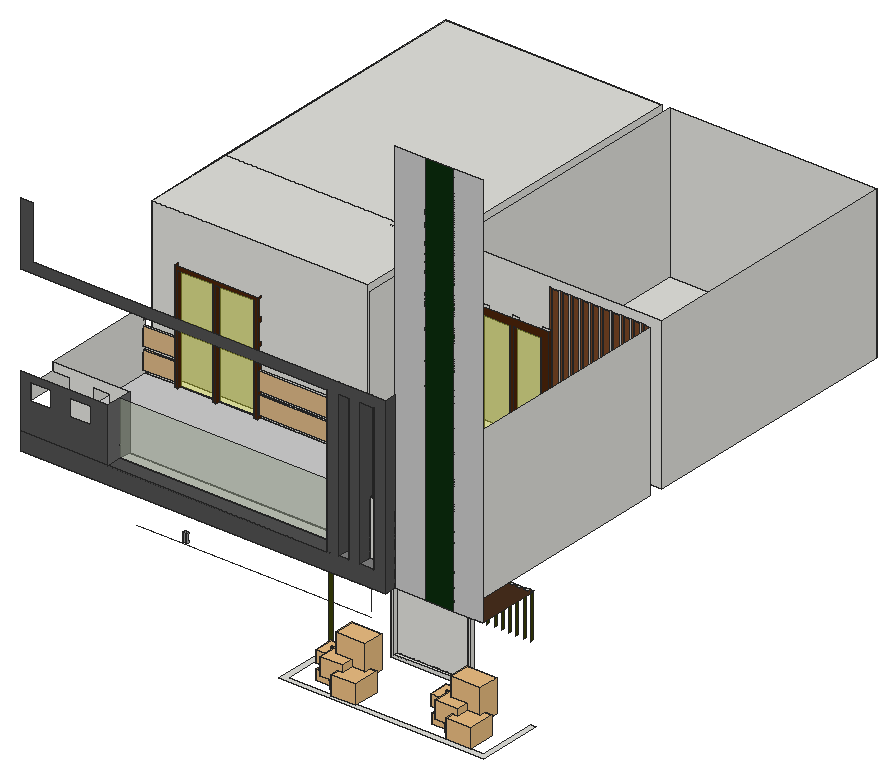
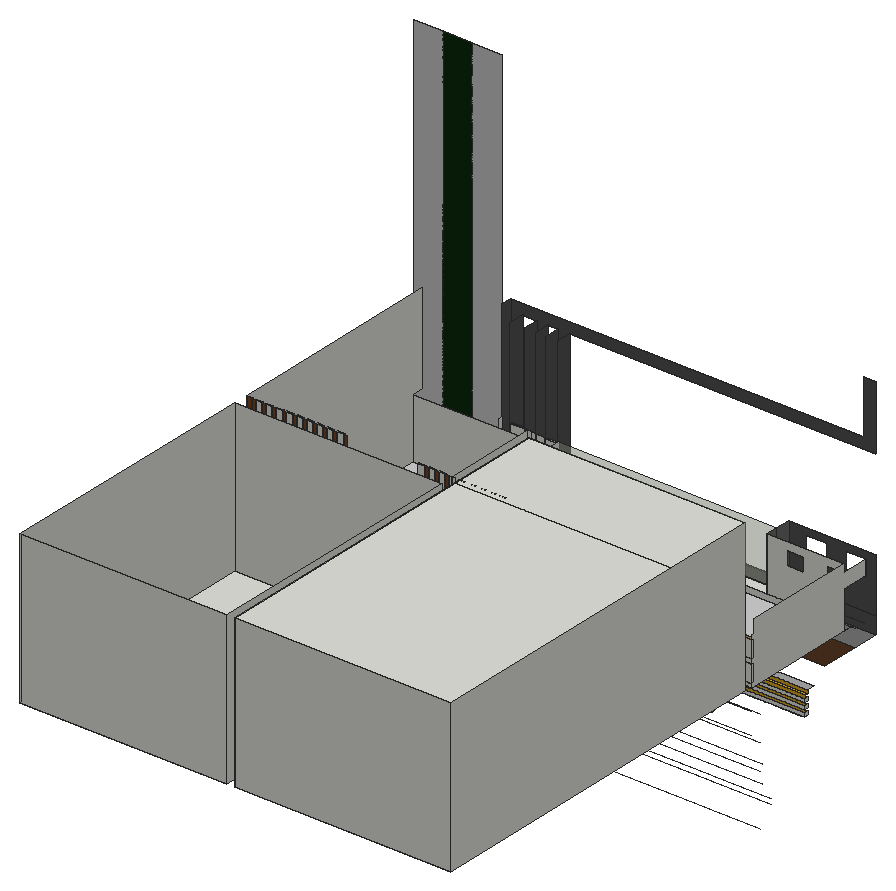
# SketchUp Ruby script. Lengths in inches.
U = 1.inch
M = Sketchup.active_model
def pt(a) = Geom::Point3d.new(a.map { |v| v * U })
def face(e, loops, mat)
  f = e.add_face(loops[0].map { |a| pt(a) })
  loops[1..].each { |l| e.add_face(l.map { |a| pt(a) }).erase! }
  f.material = f.back_material = mat if mat
  f
end
# faces: each face lists its corners as indices into pts; further lists are holes
def faces(e, pts, list, mat = nil) = list.each { |f| face(e, (f[0].is_a?(Array) ? f : [f]).map { |l| l.map { |i| pts[i] } }, mat) }
# xy, xz, yz: faces in a plane at the given z, y or x. An outline is a flat list of corners, or four numbers for a rectangle; further outlines are holes
def ring(l) = l.size == 4 ? [[l[0], l[1]], [l[2], l[1]], [l[2], l[3]], [l[0], l[3]]] : l.each_slice(2).to_a
def flat(e, list, mat, &to3) = list.each { |f| face(e, (f[0].is_a?(Array) ? f : [f]).map { |l| ring(l).map { |u, v| to3.(u, v) } }, mat) }
def xy(e, z, list, mat = nil) = flat(e, list, mat) { |x, y| [x, y, z] }
def xz(e, y, list, mat = nil) = flat(e, list, mat) { |x, z| [x, y, z] }
def yz(e, x, list, mat = nil) = flat(e, list, mat) { |y, z| [x, y, z] }
def lines(e, pts, list) = list.each { |a, b| e.add_line(pt(pts[a]), pt(pts[b])) }
# prism: a flat outline (further loops are holes) pulled along v
def prism(e, loops, v, mat = nil)
  f = face(e, loops, mat); d = Geom::Vector3d.new(v.map { |x| x * U })
  f.pushpull(f.normal.samedirection?(d) ? d.length : -d.length)
end
def box(e, o, s, mat = nil) = prism(e, [[o, [o[0] + s[0], o[1], o[2]], [o[0] + s[0], o[1] + s[1], o[2]], [o[0], o[1] + s[1], o[2]]]], [0, 0, s[2]], mat)
def at(x, y, z, deg = 0) = Geom::Transformation.translation(pt([x, y, z])) * Geom::Transformation.rotation(ORIGIN, Z_AXIS, deg.degrees)
def axes(o, x, y, z) = Geom::Transformation.new([*x, 0, *y, 0, *z, 0, *pt(o).to_a, 1])
def part(name) = M.definitions.add(name)
# library, detail: a bought-in or finely detailed component or shape, given as its bounding box
def library(name, o, s) = part(name).tap { |d| box(d.entities, o, s) }
def detail(e, o, s) = box(e.add_group.entities, o, s)
def put(e, d, t, mat = nil) = e.add_instance(d, t).tap { |i| i.material = mat if mat }
def group(e, t, mat = nil) = e.add_group.tap { |g| g.transformation = t; g.material = mat if mat }.entities
root = M.entities
M.materials.add("Material__1").color = [95, 70, 46]
M.materials.add("Material__2").color = [150, 168, 104]
M.materials.add("Material__3").color = [234, 233, 231]
M.materials.add("Material__4").color = [36, 36, 36]
M.materials.add("Material__5").color = [151, 172, 33]
M.materials.add("Material__6").color = [79, 108, 5]
M.materials.add("[0036_BurlyWood]").color = [222, 184, 135]
M.materials.add("[0043_SaddleBrown]1").color = [58, 63, 9]
M.materials.add("[0043_SaddleBrown]2").color = [76, 37, 10]
M.materials.add("[0045_Goldenrod]").color = [218, 165, 32]
M.materials.add("[0132_LightGray]").color = [169, 169, 169]
M.materials.add("[0133_Gray]").color = [128, 128, 128]
M.materials.add("[0134_DimGray]").color = [105, 105, 105]
M.materials.add("[0135_DarkGray]").color = [81, 81, 81]
M.materials.add("[Beadboard]").color = [71, 46, 29]
M.materials.add("[Carrera Marble]").color = [207, 207, 207]
M.materials.add("[Checker Plate]").color = [201, 201, 201]
M.materials.add("[Color M05]").color = [114, 114, 114]
M.materials.add("[Herringbone 4x1]").color = [12, 45, 14]
M.materials.add("[Polished Concrete Old]").color = [168, 168, 168]
M.materials.add("[Translucent Glass Blue]").color = [178, 191, 166]
M.materials["[Translucent Glass Blue]"].alpha = 0.5
M.materials.add("[Translucent Glass Gray]").color = [209, 214, 54]
M.materials["[Translucent Glass Gray]"].alpha = 0.5
M.materials.add("[Wood Veneer 01]").color = [120, 70, 37]
M.materials.add("wire_1").color = [140, 184, 58]
M.materials.add("wire_2").color = [244, 244, 244]
M.materials.add("wire_4").color = [86, 225, 198]
M.materials.add("wire_5").color = [232, 232, 232]
c1 = library("Group\#1",[-915.9375,-34.5,735.6],[41.04,40.85,6.81])
c2 = library("Group\#2",[-991.92,-34.05,729.49],[10.64,7.28,57.53])
c3 = library("Group\#3",[-1022.2,-71.69,736.68],[86.94,78.77,45.64])
c4 = library("Group\#4",[-877.77,-100.41,669.81],[37.9,37.9,42.75])
c5 = library("Group\#5",[-957.79,-83.08,701.98],[44.29,44.29,27.78])
c6 = library("Group\#6",[-1023.9,-65.47,669.625],[67.53,67.55,39.17])
c7 = library("Group\#7",[-997.48,-49.45,708.79],[29.81,29.81,30.61])
c8 = library("Group\#8",[-956738.95,-82059.81,669752.625],[42194.58,42232.57,49521.48])
c9 = library("Group\#9",[-917.52,-36.6875,711.84],[44.99,44.98,28.22])
c10 = library("Group\#10",[-916244.63,-35413.97,669800.48],[42442.38,42642.99,59706.29])
c11 = library("Group\#11",[-955.48,-54.29,730.4],[118.63,83.7,130.4])
c12 = library("Group\#12",[-899.97,-18.72,732.17],[8.78,8.27,28.64])
c13 = library("Group\#13",[-906.16,-138.28,686.8],[98.25,106.18,75.79])
c14 = library("Group\#14",[-978.71,-103.24,719.12],[90.2,76.4,68.29])
c15 = library("Group\#15",[-955.98,-81.17,725.57],[41.03,40.85,6.81])
c16 = library("Group\#16",[-996.8,-48.73,736.67],[28.51,28.38,4.73])
c17 = library("Group\#17",[-876.58,-99.29,706.19],[35.74,35.58,5.93])
c18 = library("Group\#18",[-912.1,-32.49,735.82],[33.14,36.63,9.55])
c19 = library("Group\#19",[-994.36,-46.95,735.88],[24.38,25.9,6.88])
c20 = part("PLANT-30")
p = [[0,0,0],[1,0,0],[1,1,0]]
lines(c20.entities,p,[[0,1],[1,2],[2,0]])
put(c20.entities,c1,at(895.63,-7.06,-669.82),"Material__1")
put(c20.entities,c2,at(895.63,-7.06,-669.82),"wire_1")
put(c20.entities,c3,at(895.63,-7.06,-669.82),"Material__2")
put(c20.entities,c4,at(895.63,-7.06,-669.82),"wire_2")
put(c20.entities,c5,at(895.63,-7.06,-669.82),"wire_2")
put(c20.entities,c6,at(895.63,-7.06,-669.82),"Material__3")
put(c20.entities,c7,at(895.63,-7.06,-669.82),"wire_2")
put(c20.entities,c8,axes([895.63,-7.06,-669.82],[0.001,0,0],[0,0.001,0],[0,0,0.001]),"Material__4")
put(c20.entities,c9,at(895.63,-7.06,-669.82),"wire_2")
put(c20.entities,c10,axes([895.63,-7.06,-669.82],[0.001,0,0],[0,0.001,0],[0,0,0.001]),"Material__4")
put(c20.entities,c11,at(895.63,-7.06,-669.82),"Material__5")
put(c20.entities,c12,at(895.63,-7.06,-669.82),"wire_4")
put(c20.entities,c13,at(895.63,-7.06,-669.82),"Material__6")
put(c20.entities,c14,at(895.63,-7.06,-669.82),"Material__4")
put(c20.entities,c15,at(895.63,-7.06,-669.82),"Material__1")
put(c20.entities,c16,at(895.63,-7.06,-669.82),"Material__1")
put(c20.entities,c17,at(895.63,-7.06,-669.82),"Material__1")
put(c20.entities,c18,at(895.63,-7.06,-669.82),"wire_5")
put(c20.entities,c19,at(895.63,-7.06,-669.82),"wire_5")
xy(root,15,[[198.375,17.5625,361.1875,17.5625,361.1875,68.9375,357.51,68.9375,357.51,22.19,202.875,22.19,202.875,67,198.375,67]])
xy(root,26.18,[[248.25,66,248.25,67,248.86,67,248.86,69,250.875,69,250.875,67,254.11,67,254.11,69,256.125,69,256.125,67,259.36,67,259.36,69,261.375,69,261.375,67,264.61,67,264.61,69,266.625,69,266.625,67,269.86,67,269.86,69,271.875,69,271.875,67,275.11,67,275.11,69,277.125,69,277.125,67,280.36,67,280.36,69,282.375,69,282.375,67,285.61,67,285.61,69,287.625,69,287.625,67,290.86,67,290.86,69,292.875,69,292.875,67,296.11,67,296.11,69,298.125,69,298.125,67,301.36,67,301.36,69,303.375,69,303.375,67,306.61,67,306.61,69,308.625,69,308.625,67,311.86,67,311.86,69,312.4375,69,312.4375,66],[248.25,67,248.86,69],[250.875,67,254.11,69],[256.125,67,259.36,69],[261.375,67,264.61,69],
  [266.625,67,269.86,69],[271.875,67,275.11,69],[277.125,67,280.36,69],[282.375,67,285.61,69],[287.625,67,290.86,69],
  [292.875,67,296.11,69],[298.125,67,301.36,69],[303.375,67,306.61,69],[308.625,67,311.86,69]])
xy(root,29.18,[[251.25,66,309.4375,69]])
xy(root,51.4,[[85.07,64,85.08,65],[85.07,65,85.08,66]])
xy(root,51.4,[[85.08,64,85.45,66],[87.63,64,88.01,66]],"[0132_LightGray]")
xy(root,52.46,[[85.07,65,85.08,66]])
xy(root,52.46,[[85.08,65,85.45,66],[87.63,65,88.01,66]],"[0132_LightGray]")
xy(root,57.65,[[85.44,65,85.45,66]])
xy(root,57.65,[[85.07,65,85.44,66],[87.63,65,88.01,66]],"[0132_LightGray]")
xy(root,58.71,[[85.07,64,85.08,65],[85.08,64,85.44,65],[85.44,64,85.45,65],[85.07,65,85.44,66],[85.44,65,85.45,66]])
xy(root,58.71,[[87.63,64,88.01,66]],"[0132_LightGray]")
xy(root,75.79,[[8.86,66,8.86,67,12.35,67,12.35,69,14.55,69,14.55,67,18.04,67,18.04,69,20.24,69,20.24,67,23.72,67,23.72,69,25.93,69,25.93,67,29.41,67,29.41,69,31.61,69,31.61,67,35.1,67,35.1,69,37.3,69,37.3,67,40.79,67,40.79,69,42.99,69,42.99,67,46.47,67,46.47,69,48.68,69,48.68,67,52.16,67,52.16,69,54.36,69,54.36,67,57.85,67,57.85,69,60.05,69,60.05,67,63.54,67,63.54,69,65.74,69,65.74,67,69.22,67,69.22,69,71.43,69,71.43,67,74.91,67,74.91,69,76.57,69,76.57,66],[76.57,66,85.45,69],[85.45,66,87.63,69],[87.63,66,96.52,69],[96.52,66,96.52,69,97.66,69,97.66,67,99.86,67,99.86,69,103.35,69,103.35,67,105.55,67,105.55,69,109.04,69,109.04,67,111.24,67,111.24,69,114.72,69,114.72,67,116.93,67,116.93,69,120.41,69,120.41,67,122.61,67,122.61,69,126.1,69,126.1,67,128.3,67,128.3,69,131.79,69,131.79,67,133.99,67,133.99,69,137.47,69,137.47,67,139.68,67,139.68,69,143.16,69,143.16,67,145.36,67,145.36,69,148.85,69,148.85,67,151.05,67,151.05,69,154.54,69,154.54,67,156.74,67,156.74,69,160.22,69,160.22,67,162.43,67,162.43,69,165.91,69,165.91,67,168.11,67,168.11,69,171.6,69,171.6,67,173.8,67,173.8,69,177.29,69,177.29,67,179.49,67,179.49,69,182.97,69,182.97,67,184.43,67,184.43,66],
  [8.86,67,12.35,69],[14.55,67,18.04,69],[20.24,67,23.72,69],[25.93,67,29.41,69],[31.61,67,35.1,69],
  [37.3,67,40.79,69],[42.99,67,46.47,69],[48.68,67,52.16,69],[54.36,67,57.85,69],[60.05,67,63.54,69],
  [65.74,67,69.22,69],[71.43,67,74.91,69],[97.66,67,99.86,69],[103.35,67,105.55,69],[109.04,67,111.24,69],
  [114.72,67,116.93,69],[120.41,67,122.61,69],[126.1,67,128.3,69],[131.79,67,133.99,69],[137.47,67,139.68,69],
  [143.16,67,145.36,69],[148.85,67,151.05,69],[154.54,67,156.74,69],[160.22,67,162.43,69],[165.91,67,168.11,69],
  [171.6,67,173.8,69],[177.29,67,179.49,69],[182.97,67,184.43,69]])
xy(root,78.7,[[8.86,66,184.43,69]],"[0045_Goldenrod]")
xy(root,80.98,[[8.86,66,184.43,69]],"[0045_Goldenrod]")
xy(root,81.93,[[251.25,66,309.4375,69]])
xy(root,83.88,[[8.86,66,184.43,69]],"[0045_Goldenrod]")
xy(root,84.93,[[248.25,66,312.4375,66,312.4375,69,311.86,69,311.86,67,308.625,67,308.625,69,306.61,69,306.61,67,303.375,67,303.375,69,301.36,69,301.36,67,298.125,67,298.125,69,296.11,69,296.11,67,292.875,67,292.875,69,290.86,69,290.86,67,287.625,67,287.625,69,285.61,69,285.61,67,282.375,67,282.375,69,280.36,69,280.36,67,277.125,67,277.125,69,275.11,69,275.11,67,271.875,67,271.875,69,269.86,69,269.86,67,266.625,67,266.625,69,264.61,69,264.61,67,261.375,67,261.375,69,259.36,69,259.36,67,256.125,67,256.125,69,254.11,69,254.11,67,250.875,67,250.875,69,248.86,69,248.86,67,248.25,67],[248.25,67,248.86,69],[250.875,67,254.11,69],[256.125,67,259.36,69],[261.375,67,264.61,69],
  [266.625,67,269.86,69],[271.875,67,275.11,69],[277.125,67,280.36,69],[282.375,67,285.61,69],[287.625,67,290.86,69],
  [292.875,67,296.11,69],[298.125,67,301.36,69],[303.375,67,306.61,69],[308.625,67,311.86,69]])
xy(root,86.17,[[8.86,66,184.43,69]],"[0045_Goldenrod]")
xy(root,89.07,[[8.86,66,184.43,69]],"[0045_Goldenrod]")
xy(root,91.35,[[8.86,66,184.43,69]],"[0045_Goldenrod]")
xy(root,94.26,[[8.86,60,184.43,66]],"[Polished Concrete Old]")
xy(root,111.13,[[198.375,67,201.61,69],[203.625,67,206.86,69],[208.875,67,212.11,69],[214.125,67,217.36,69],[219.375,67,222.61,69],
  [224.625,67,227.86,69],[229.875,67,233.11,69],[235.125,67,238.36,69],[240.375,67,243.61,69],[245.625,67,248.86,69],
  [250.875,67,254.11,69],[256.125,67,259.36,69],[261.375,67,264.61,69],[266.625,67,269.86,69],[271.875,67,275.11,69],
  [277.125,67,280.36,69],[282.375,67,285.61,69],[287.625,67,290.86,69],[292.875,67,296.11,69],[298.125,67,301.36,69],
  [303.375,67,306.61,69],[308.625,67,311.86,69],[313.875,67,317.11,69],[319.125,67,322.36,69],[324.375,67,327.61,69],
  [330.125,67,333.36,69],[335.875,67,339.11,69],[341.625,67,344.86,69],[347.375,67,350.61,69],[353.125,67,356.36,69],
  [358.875,67,360,69],[219.375,69,222.61,265.8125]])
xy(root,111.13,[[290.11,18,290.11,30,0,30,0,60,193.125,60,193.125,67,196.36,67,196.36,69,198.375,69,198.375,67,201.61,67,201.61,69,203.625,69,203.625,67,206.86,67,206.86,69,208.875,69,208.875,67,212.11,67,212.11,69,214.125,69,214.125,67,217.36,67,217.36,69,219.375,69,219.375,67,222.61,67,222.61,69,224.625,69,224.625,67,227.86,67,227.86,69,229.875,69,229.875,67,233.11,67,233.11,69,235.125,69,235.125,67,238.36,67,238.36,69,240.375,69,240.375,67,243.61,67,243.61,69,245.625,69,245.625,67,248.86,67,248.86,69,250.875,69,250.875,67,254.11,67,254.11,69,256.125,69,256.125,67,259.36,67,259.36,69,261.375,69,261.375,67,264.61,67,264.61,69,266.625,69,266.625,67,269.86,67,269.86,69,271.875,69,271.875,67,275.11,67,275.11,69,277.125,69,277.125,67,280.36,67,280.36,69,282.375,69,282.375,67,285.61,67,285.61,69,287.625,69,287.625,67,290.86,67,290.86,69,292.875,69,292.875,67,296.11,67,296.11,69,298.125,69,298.125,67,301.36,67,301.36,69,303.375,69,303.375,67,306.61,67,306.61,69,308.625,69,308.625,67,311.86,67,311.86,69,313.875,69,313.875,67,317.11,67,317.11,69,319.125,69,319.125,67,322.36,67,322.36,69,324.375,69,324.375,67,327.61,67,327.61,69,330.125,69,330.125,67,333.36,67,333.36,69,335.875,69,335.875,67,339.11,67,339.11,69,341.625,69,341.625,67,344.86,67,344.86,69,347.375,69,347.375,67,350.61,67,350.61,69,353.125,69,353.125,67,356.36,67,356.36,69,358.875,69,358.875,67,360,67,360,18]],"[Beadboard]")
xy(root,111.13,[[0,9,290.11,30]],"[Color M05]")
xy(root,120,[[34.44,118.875,37.44,121.875],[64.75,118.875,67.75,121.875],[97.44,118.875,100.44,121.875],[9,127.875,180.9375,420],[212.08,193.3125,218.08,196.3125],
  [241.58,193.3125,244.58,196.3125],[266.08,193.3125,272.08,196.3125],[192.78,195.3125,197.8125,196.3125],[200.84,195.3125,205.875,196.3125],[208.9,195.3125,212.08,196.3125],
  [273.4,195.3125,278.4375,196.3125],[281.47,195.3125,286.5,196.3125],[289.53,195.3125,294.5625,196.3125],[297.59,195.3125,302.625,196.3125],[305.65,195.3125,310.6875,196.3125],
  [313.72,195.3125,318.75,196.3125],[321.78,195.3125,326.8125,196.3125],[329.84,195.3125,334.875,196.3125],[337.9,195.3125,342.9375,196.3125],[186.9375,196,189.75,196.3125],
  [186.9375,207,351,420]])
xy(root,120,[[8.88,30,351,30,351,195.3125,345.97,195.3125,345.97,196.3125,342.9375,196.3125,342.9375,195.3125,337.9,195.3125,337.9,196.3125,334.875,196.3125,334.875,195.3125,329.84,195.3125,329.84,196.3125,326.8125,196.3125,326.8125,195.3125,321.78,195.3125,321.78,196.3125,318.75,196.3125,318.75,195.3125,313.72,195.3125,313.72,196.3125,310.6875,196.3125,310.6875,195.3125,305.65,195.3125,305.65,196.3125,302.625,196.3125,302.625,195.3125,297.59,195.3125,297.59,196.3125,294.5625,196.3125,294.5625,195.3125,289.53,195.3125,289.53,196.3125,286.5,196.3125,286.5,195.3125,281.47,195.3125,281.47,196.3125,278.4375,196.3125,278.4375,195.3125,273.4,195.3125,273.4,196.3125,272.08,196.3125,272.08,193.3125,266.08,193.3125,266.08,196.3125,244.58,196.3125,244.58,193.3125,241.58,193.3125,241.58,196.3125,218.08,196.3125,218.08,193.3125,212.08,193.3125,212.08,195.3125,208.9,195.3125,208.9,196.3125,205.875,196.3125,205.875,195.3125,200.84,195.3125,200.84,196.3125,197.8125,196.3125,197.8125,195.3125,192.78,195.3125,192.78,196.3125,189.75,196.3125,189.75,196,186.9375,196,186.9375,121.875,100.44,121.875,100.44,118.875,97.44,118.875,97.44,121.875,67.75,121.875,67.75,118.875,64.75,118.875,64.75,121.875,37.44,121.875,37.44,118.875,34.44,118.875,34.44,121.875,8.88,121.875]],"[Carrera Marble]")
xy(root,123.05,[[8.88,119.875,34.44,121.875],[100.44,119.875,186.9375,121.875]])
xy(root,124.86,[[243.73,9,252.65,21],[260.55,9,269.46,21],[269.46,19.25,281.11,19.625],[269.46,19.625,281.11,21],[69.79,21,242.89,30],
  [242.89,21,243.73,21,243.73,22.5625,243.52,22.5625,243.52,30,242.89,30],[243.73,21,252.65,22.5625],[243.52,22.5625,243.73,30]])
xy(root,124.86,[[252.65,9,260.55,21],[269.46,9,281.11,19.25]],"[0133_Gray]")
xy(root,124.86,[[69.79,9,243.73,21]],"[0135_DarkGray]")
xy(root,137.25,[[8.88,119.875,9,121.875],[100.44,119.875,186.9375,121.875]])
xy(root,137.25,[[9,119.875,34.44,121.875]],"[0036_BurlyWood]")
xy(root,140.17,[[8.88,119.875,34.44,121.875],[100.44,119.875,186.9375,121.875]])
xy(root,240,[[9,127.875,180.9375,201],[9,201,180.9375,420]])
xz(root,9,[[[0,111.13,290.11,111.13,290.11,248.55,9.76,248.55,9.76,291,0,291,0,240,243.73,240,243.73,124.86,0,124.86],[269.46,124.86,281.11,240],[252.65,124.86,260.55,240]],[[0,124.86,69.79,168],[7.61,149,23.86,162.68],[39.61,149,55.86,162.68]]],"[0135_DarkGray]")
xz(root,18,[[290.11,111.13,314.22,426],[337.25,111.13,360,426]],"[Checker Plate]")
xz(root,18,[[314.22,111.13,337.25,426]],"[Herringbone 4x1]")
xz(root,19.25,[[269.46,124.86,281.11,168]])
xz(root,19.625,[[269.46,124.86,281.11,168]])
xz(root,21,[[242.89,124.86,243.73,168],[243.73,124.86,252.65,168],[252.65,124.86,260.55,168.11],[260.55,124.86,263.86,168],[263.86,124.86,269.46,168],
  [269.46,124.86,281.11,168]])
xz(root,21,[[69.79,124.86,242.89,168.11]],"[Translucent Glass Blue]")
xz(root,22.5625,[[243.52,124.86,243.73,168],[243.73,124.86,252.65,168]])
xz(root,30,[[8.88,120,8.88,124.86,242.89,124.86,242.89,168.11,281.11,168.11,281.11,168,351,168,351,120],[[8.88,124.86,8.88,150.27,22.59,150.27,22.59,161.41,8.88,161.41,8.88,168,69.79,168,69.79,124.86],[40.88,150.27,54.59,161.41]]])
xz(root,64,[[85.07,51.4,85.45,58.71],[87.63,51.4,88.01,58.71]],"[0132_LightGray]")
xz(root,65,[[85.07,52.46,85.08,57.65],[85.08,52.46,85.45,57.65],[87.63,52.46,88.01,57.65]])
xz(root,66,[[[248.25,26.18,312.4375,84.93],[251.25,29.18,309.4375,81.93]],[85.07,51.4,85.08,52.46],[85.08,51.4,85.45,52.46],[87.63,51.4,88.01,52.46],[85.07,57.65,85.44,58.71],
  [85.44,57.65,85.45,58.71],[87.63,57.65,88.01,58.71]])
xz(root,66,[[8.86,75.79,184.43,78.7],[8.86,80.98,184.43,83.88],[8.86,86.17,184.43,89.07],[8.86,91.35,184.43,94.26]],"[0045_Goldenrod]")
xz(root,67,[[198.375,15,201.61,111.13],[250.875,84.93,254.11,111.13],[256.125,84.93,259.36,111.13],[261.375,84.93,264.61,111.13],[266.625,84.93,269.86,111.13],
  [271.875,84.93,275.11,111.13],[277.125,84.93,280.36,111.13],[282.375,84.93,285.61,111.13],[287.625,84.93,290.86,111.13],[292.875,84.93,296.11,111.13],
  [298.125,84.93,301.36,111.13],[303.375,84.93,306.61,111.13],[308.625,84.93,311.86,111.13]],"[0043_SaddleBrown]1")
xz(root,69,[[248.25,26.18,248.86,84.93],[250.875,26.18,254.11,26.18,254.11,29.18,251.25,29.18,251.25,81.93,254.11,81.93,254.11,84.93,250.875,84.93],[256.125,26.18,259.36,29.18],[261.375,26.18,264.61,29.18],[266.625,26.18,269.86,29.18],
  [271.875,26.18,275.11,29.18],[277.125,26.18,280.36,29.18],[282.375,26.18,285.61,29.18],[287.625,26.18,290.86,29.18],[292.875,26.18,296.11,29.18],
  [298.125,26.18,301.36,29.18],[303.375,26.18,306.61,29.18],[308.625,26.18,311.86,26.18,311.86,84.93,308.625,84.93,308.625,81.93,309.4375,81.93,309.4375,29.18,308.625,29.18],[251.25,29.18,309.4375,81.93],[8.86,75.79,184.43,78.7],
  [8.86,80.98,184.43,83.88],[256.125,81.93,259.36,84.93],[261.375,81.93,264.61,84.93],[266.625,81.93,269.86,84.93],[271.875,81.93,275.11,84.93],
  [277.125,81.93,280.36,84.93],[282.375,81.93,285.61,84.93],[287.625,81.93,290.86,84.93],[292.875,81.93,296.11,84.93],[298.125,81.93,301.36,84.93],
  [303.375,81.93,306.61,84.93],[248.86,84.93,250.875,111.13],[250.875,84.93,254.11,111.13],[254.11,84.93,256.125,111.13],[256.125,84.93,259.36,111.13],
  [259.36,84.93,261.375,111.13],[261.375,84.93,264.61,111.13],[264.61,84.93,266.625,111.13],[266.625,84.93,269.86,111.13],[269.86,84.93,271.875,111.13],
  [271.875,84.93,275.11,111.13],[275.11,84.93,277.125,111.13],[277.125,84.93,280.36,111.13],[280.36,84.93,282.375,111.13],[282.375,84.93,285.61,111.13],
  [285.61,84.93,287.625,111.13],[287.625,84.93,290.86,111.13],[290.86,84.93,292.875,111.13],[292.875,84.93,296.11,111.13],[296.11,84.93,298.125,111.13],
  [298.125,84.93,301.36,111.13],[301.36,84.93,303.375,111.13],[303.375,84.93,306.61,111.13],[306.61,84.93,308.625,111.13],[308.625,84.93,311.86,111.13],
  [8.86,86.17,184.43,89.07]])
xz(root,69,[[8.86,78.7,184.43,80.98],[8.86,83.88,184.43,86.17],[8.86,89.07,184.43,91.35]],"[0045_Goldenrod]")
xz(root,118.875,[[34.44,120,37.44,120,37.44,204,64.75,204,64.75,120,67.75,120,67.75,204,97.44,204,97.44,120,100.44,120,100.44,207,34.44,207]],"[0043_SaddleBrown]2")
xz(root,119.875,[[8.88,123.05,34.44,137.25],[100.44,123.05,186.9375,137.25],[8.88,140.17,34.44,154.375],[100.44,140.17,186.9375,154.375]],"[0036_BurlyWood]")
xz(root,121.875,[[34.44,117,100.44,120],[34.44,117,100.44,120],[8.88,120,34.44,120.125],[34.44,120,37.44,120.125],[37.44,120,64.75,120.125],
  [64.75,120,67.75,120.125],[67.75,120,97.44,120.125],[97.44,120,100.44,120.125],[100.44,120,186.9375,120.125],[8.88,120.125,34.44,123.05],
  [34.44,120.125,37.44,123.05],[64.75,120.125,67.75,123.05],[97.44,120.125,100.44,123.05],[100.44,120.125,186.9375,123.05],[8.88,123.05,34.44,137.25],
  [34.44,123.05,37.44,137.25],[64.75,123.05,67.75,137.25],[97.44,123.05,100.44,137.25],[100.44,123.05,186.9375,137.25],[8.88,137.25,34.44,140.17],
  [34.44,137.25,37.44,140.17],[64.75,137.25,67.75,140.17],[97.44,137.25,100.44,140.17],[100.44,137.25,186.9375,140.17],[8.88,140.17,34.44,154.375],
  [34.44,140.17,37.44,154.375],[64.75,140.17,67.75,154.375],[97.44,140.17,100.44,154.375],[100.44,140.17,186.9375,154.375]])
xz(root,121.875,[[37.44,120.125,64.75,204],[67.75,120.125,97.44,204]],"[Translucent Glass Gray]")
xz(root,127.875,[[9,120,180.9375,240]])
xz(root,193.3125,[[212.08,120,218.08,120,218.08,204,241.58,204,241.58,120,244.58,120,244.58,204,266.08,204,266.08,120,272.08,120,272.08,210,212.08,210]],"[0043_SaddleBrown]2")
xz(root,195.3125,[[192.78,120,197.8125,240],[200.84,120,205.875,240],[208.9,120,212.08,120,212.08,210,213.9375,210,213.9375,240,208.9,240],[273.4,120,278.4375,240],[281.47,120,286.5,240],
  [289.53,120,294.5625,240],[297.59,120,302.625,240],[305.65,120,310.6875,240],[313.72,120,318.75,240],[321.78,120,326.8125,240],
  [329.84,120,334.875,240],[337.9,120,342.9375,240],[345.97,120,351,240]],"[Wood Veneer 01]")
xz(root,196,[[186.9375,120,189.75,240]],"[Wood Veneer 01]")
xz(root,196.3125,[[212.08,114,272.08,120],[144.4,120,149.4375,240],[152.47,120,157.5,240],[160.53,120,165.5625,240],[168.59,120,173.625,240],
  [176.65,120,181.6875,240],[184.72,120,186.9375,240],[186.9375,120,189.75,240],[192.78,120,197.8125,240],[200.84,120,205.875,240],
  [208.9,120,208.9,240,213.9375,240,213.9375,210,212.08,210,212.08,120],[212.08,120,213.9375,210],[213.9375,120,216.97,210],[216.97,120,218.08,120,218.08,204,222,204,222,210,216.97,210],[241.58,120,244.58,120,244.58,204,246.1875,204,246.1875,210,241.15,210,241.15,204,241.58,204],
  [266.08,120,270.375,120,270.375,210,265.34,210,265.34,204,266.08,204],[270.375,120,272.08,210],[273.4,120,278.4375,240],[281.47,120,286.5,240],[289.53,120,294.5625,240],
  [297.59,120,302.625,240],[305.65,120,310.6875,240],[313.72,120,318.75,240],[321.78,120,326.8125,240],[329.84,120,334.875,240],
  [337.9,120,342.9375,240]])
xz(root,196.3125,[[218.08,120,241.58,204],[244.58,120,266.08,204]],"[Translucent Glass Gray]")
xz(root,196.3125,[[189.75,120,192.78,240],[197.8125,120,200.84,240],[205.875,120,208.9,240],[272.08,120,273.4,120,273.4,240,270.375,240,270.375,210,272.08,210],[278.4375,120,281.47,240],
  [286.5,120,289.53,240],[294.5625,120,297.59,240],[302.625,120,305.65,240],[310.6875,120,313.72,240],[318.75,120,321.78,240],
  [326.8125,120,329.84,240],[334.875,120,337.9,240],[342.9375,120,345.97,240]],"[Wood Veneer 01]")
xz(root,207,[[186.9375,120,351,240]])
xz(root,420,[[9,120,180.9375,240],[186.9375,120,351,240]])
yz(root,8.86,[[66,75.79,69,78.7],[66,80.98,69,83.88],[66,86.17,69,89.07]])
yz(root,8.88,[[30,120,121.875,120,121.875,123.05,119.875,123.05,119.875,137.25,121.875,137.25,121.875,140.17,119.875,140.17,119.875,154.375,121.875,154.375,121.875,157.3,119.875,157.3,119.875,168.11,30,168.11,30,161.41,9,161.41,9,150.27,30,150.27],[119.875,123.05,121.875,137.25],[119.875,140.17,121.875,154.375]])
yz(root,9,[[127.875,120,420,240]])
yz(root,34.44,[[119.875,123.05,121.875,137.25],[119.875,140.17,121.875,154.375]])
yz(root,34.44,[[118.875,120,118.875,207,121.875,207,121.875,205.75,119.875,205.75,119.875,191.55,121.875,191.55,121.875,188.625,119.875,188.625,119.875,174.42,121.875,174.42,121.875,171.5,119.875,171.5,119.875,157.3,121.875,157.3,121.875,154.375,119.875,154.375,119.875,140.17,121.875,140.17,121.875,137.25,119.875,137.25,119.875,123.05,121.875,123.05,121.875,120]],"[0043_SaddleBrown]2")
yz(root,37.44,[[118.875,120,121.875,204]],"[0043_SaddleBrown]2")
yz(root,64.75,[[118.875,120,121.875,204]],"[0043_SaddleBrown]2")
yz(root,67.75,[[118.875,120,121.875,204]],"[0043_SaddleBrown]2")
yz(root,69.79,[[9,124.86,21,168],[21,124.86,30,168]],"[0134_DimGray]")
yz(root,85.07,[[64,51.4,64,58.71,66,58.71,66,57.65,65,57.65,65,52.46,66,52.46,66,51.4]],"[0132_LightGray]")
yz(root,85.45,[[64,51.4,66,51.4,66,52.46,65,52.46,65,57.65,66,57.65,66,58.71,64,58.71]],"[0132_LightGray]")
yz(root,87.63,[[64,51.4,64,58.71,66,58.71,66,57.65,65,57.65,65,52.46,66,52.46,66,51.4]],"[0132_LightGray]")
yz(root,88.01,[[64,51.4,66,51.4,66,52.46,65,52.46,65,57.65,66,57.65,66,58.71,64,58.71]],"[0132_LightGray]")
yz(root,97.44,[[118.875,120,121.875,204]],"[0043_SaddleBrown]2")
yz(root,100.44,[[119.875,123.05,121.875,137.25],[119.875,140.17,121.875,154.375]])
yz(root,100.44,[[118.875,120,121.875,120,121.875,123.05,119.875,123.05,119.875,137.25,121.875,137.25,121.875,140.17,119.875,140.17,119.875,154.375,121.875,154.375,121.875,157.3,119.875,157.3,119.875,171.5,121.875,171.5,121.875,174.42,119.875,174.42,119.875,188.625,121.875,188.625,121.875,191.55,119.875,191.55,119.875,205.75,121.875,205.75,121.875,207,118.875,207]],"[0043_SaddleBrown]2")
yz(root,180.9375,[[127.875,120,420,240]])
yz(root,184.43,[[66,75.79,69,78.7],[66,80.98,69,83.88],[66,86.17,69,89.07]])
yz(root,186.9375,[[121.875,120,196,240],[196,120,196.3125,240],[207,120,420,240],[119.875,123.05,121.875,137.25],[119.875,140.17,121.875,154.375]])
yz(root,189.75,[[196,120,196.3125,240]])
yz(root,192.78,[[195.3125,120,196.3125,240]])
yz(root,197.8125,[[195.3125,120,196.3125,240]])
yz(root,198.375,[[67,75.79,69,111.13]],"[0043_SaddleBrown]1")
yz(root,200.84,[[195.3125,120,196.3125,240]])
yz(root,203.625,[[67,75.79,69,111.13]],"[0043_SaddleBrown]1")
yz(root,205.875,[[195.3125,120,196.3125,240]])
yz(root,208.875,[[67,75.79,69,111.13]],"[0043_SaddleBrown]1")
yz(root,208.9,[[195.3125,120,196.3125,240]])
yz(root,212.08,[[193.3125,120,195.3125,210],[195.3125,120,196.3125,210]])
yz(root,214.125,[[67,75.79,69,111.13]],"[0043_SaddleBrown]1")
yz(root,218.08,[[193.3125,120,196.3125,204]],"[0043_SaddleBrown]2")
yz(root,219.375,[[69,75.79,265.8125,111.13]])
yz(root,219.375,[[67,75.79,69,111.13]],"[0043_SaddleBrown]1")
yz(root,224.625,[[67,75.79,69,111.13]],"[0043_SaddleBrown]1")
yz(root,229.875,[[67,75.79,69,111.13]],"[0043_SaddleBrown]1")
yz(root,235.125,[[67,75.79,69,111.13]],"[0043_SaddleBrown]1")
yz(root,240.375,[[67,75.79,69,111.13]],"[0043_SaddleBrown]1")
yz(root,241.58,[[193.3125,120,196.3125,204]],"[0043_SaddleBrown]2")
yz(root,242.89,[[21,124.86,30,168.11]])
yz(root,243.73,[[21,124.86,22.5625,168]])
yz(root,243.73,[[9,124.86,21,240]],"[0135_DarkGray]")
yz(root,244.58,[[193.3125,120,196.3125,204]],"[0043_SaddleBrown]2")
yz(root,245.625,[[67,75.79,69,111.13]],"[0043_SaddleBrown]1")
yz(root,248.25,[[66,26.18,67,84.93],[67,26.18,69,84.93]])
yz(root,248.86,[[67,84.93,69,111.13]],"[0043_SaddleBrown]1")
yz(root,250.875,[[67,84.93,69,111.13]],"[0043_SaddleBrown]1")
yz(root,251.25,[[66,29.18,69,81.93]])
yz(root,252.65,[[21,124.86,22.5625,168]])
yz(root,252.65,[[9,124.86,21,240]],"[0135_DarkGray]")
yz(root,254.11,[[67,84.93,69,111.13]],"[0043_SaddleBrown]1")
yz(root,256.125,[[67,84.93,69,111.13]],"[0043_SaddleBrown]1")
yz(root,259.36,[[67,84.93,69,111.13]],"[0043_SaddleBrown]1")
yz(root,260.55,[[9,124.86,21,240]],"[0135_DarkGray]")
yz(root,261.375,[[67,84.93,69,111.13]],"[0043_SaddleBrown]1")
yz(root,264.61,[[67,84.93,69,111.13]],"[0043_SaddleBrown]1")
yz(root,266.08,[[193.3125,120,196.3125,204]],"[0043_SaddleBrown]2")
yz(root,266.625,[[67,84.93,69,111.13]],"[0043_SaddleBrown]1")
yz(root,269.46,[[19.25,124.86,19.625,168],[19.625,124.86,21,168]])
yz(root,269.46,[[9,124.86,19.25,124.86,19.25,168,21,168,21,240,9,240]],"[0135_DarkGray]")
yz(root,269.86,[[67,84.93,69,111.13]],"[0043_SaddleBrown]1")
yz(root,271.875,[[67,84.93,69,111.13]],"[0043_SaddleBrown]1")
yz(root,272.08,[[193.3125,120,196.3125,210]],"[0043_SaddleBrown]2")
yz(root,273.4,[[195.3125,120,196.3125,240]],"[Wood Veneer 01]")
yz(root,275.11,[[67,84.93,69,111.13]],"[0043_SaddleBrown]1")
yz(root,277.125,[[67,84.93,69,111.13]],"[0043_SaddleBrown]1")
yz(root,278.4375,[[195.3125,120,196.3125,240]])
yz(root,280.36,[[67,84.93,69,111.13]],"[0043_SaddleBrown]1")
yz(root,281.11,[[19.25,124.86,19.625,168],[19.625,124.86,21,168]])
yz(root,281.11,[[9,124.86,9,240,21,240,21,168,19.25,168,19.25,124.86]],"[0135_DarkGray]")
yz(root,281.47,[[195.3125,120,196.3125,240]],"[Wood Veneer 01]")
yz(root,282.375,[[67,84.93,69,111.13]],"[0043_SaddleBrown]1")
yz(root,285.61,[[67,84.93,69,111.13]],"[0043_SaddleBrown]1")
yz(root,286.5,[[195.3125,120,196.3125,240]])
yz(root,287.625,[[67,84.93,69,111.13]],"[0043_SaddleBrown]1")
yz(root,289.53,[[195.3125,120,196.3125,240]],"[Wood Veneer 01]")
yz(root,290.11,[[18,111.13,21,168]])
yz(root,290.11,[[9,111.13,18,248.55]],"[0135_DarkGray]")
yz(root,290.86,[[67,84.93,69,111.13]],"[0043_SaddleBrown]1")
yz(root,292.875,[[67,84.93,69,111.13]],"[0043_SaddleBrown]1")
yz(root,294.5625,[[195.3125,120,196.3125,240]])
yz(root,296.11,[[67,84.93,69,111.13]],"[0043_SaddleBrown]1")
yz(root,297.59,[[195.3125,120,196.3125,240]],"[Wood Veneer 01]")
yz(root,298.125,[[67,84.93,69,111.13]],"[0043_SaddleBrown]1")
yz(root,301.36,[[67,84.93,69,111.13]],"[0043_SaddleBrown]1")
yz(root,302.625,[[195.3125,120,196.3125,240]])
yz(root,303.375,[[67,84.93,69,111.13]],"[0043_SaddleBrown]1")
yz(root,305.65,[[195.3125,120,196.3125,240]],"[Wood Veneer 01]")
yz(root,306.61,[[67,84.93,69,111.13]],"[0043_SaddleBrown]1")
yz(root,308.625,[[67,84.93,69,111.13]],"[0043_SaddleBrown]1")
yz(root,309.4375,[[66,29.18,69,81.93]])
yz(root,310.6875,[[195.3125,120,196.3125,240]])
yz(root,311.86,[[67,84.93,69,111.13]],"[0043_SaddleBrown]1")
yz(root,312.4375,[[66,26.18,69,84.93]])
yz(root,313.72,[[195.3125,120,196.3125,240]],"[Wood Veneer 01]")
yz(root,313.875,[[67,75.79,69,111.13]],"[0043_SaddleBrown]1")
yz(root,318.75,[[195.3125,120,196.3125,240]])
yz(root,319.125,[[67,75.79,69,111.13]],"[0043_SaddleBrown]1")
yz(root,321.78,[[195.3125,120,196.3125,240]],"[Wood Veneer 01]")
yz(root,324.375,[[67,75.79,69,111.13]],"[0043_SaddleBrown]1")
yz(root,326.8125,[[195.3125,120,196.3125,240]])
yz(root,329.84,[[195.3125,120,196.3125,240]],"[Wood Veneer 01]")
yz(root,330.125,[[67,75.79,69,111.13]],"[0043_SaddleBrown]1")
yz(root,334.875,[[195.3125,120,196.3125,240]])
yz(root,335.875,[[67,75.79,69,111.13]],"[0043_SaddleBrown]1")
yz(root,337.9,[[195.3125,120,196.3125,240]],"[Wood Veneer 01]")
yz(root,341.625,[[67,75.79,69,111.13]],"[0043_SaddleBrown]1")
yz(root,342.9375,[[195.3125,120,196.3125,240]])
yz(root,345.97,[[195.3125,120,196.3125,240]],"[Wood Veneer 01]")
yz(root,347.375,[[67,75.79,69,111.13]],"[0043_SaddleBrown]1")
yz(root,351,[[30,120,30,168.11,21,168.11,21,240,195.3125,240,195.3125,120],[207,120,420,240]])
yz(root,353.125,[[67,75.79,69,111.13]],"[0043_SaddleBrown]1")
yz(root,358.875,[[67,75.79,69,111.13]],"[0043_SaddleBrown]1")
p = [[9,30,120],[9,21,120],[351,30,120],[351,21,120],[69.79,21,124.86],[0,21,124.86],
  [281.11,21,124.86],[281.11,30,124.86],[8.88,30,124.86],[0,30,124.86],[290.11,30,120],[290.11,30,111.13],
  [252.65,22.5625,124.86],[252.65,30,124.86],[260.55,21,124.86],[260.55,30,124.86],[195.9375,112.875,101.41],[195.9375,112.875,117.75],
  [9,112.875,117.75],[195.9375,112.875,80.97],[195.9375,112.875,97.3125],[9,112.875,97.3125],[195.9375,112.875,60.53],[195.9375,112.875,76.875],
  [9,112.875,76.875],[195.9375,112.875,40.09],[0,112.875,40.09],[195.9375,112.875,56.4375],[9,112.875,56.4375],[195.9375,112.875,19.66],
  [195.9375,112.875,36],[9,112.875,36],[0,112.875,36],[9,112.875,15.5625],[195.9375,112.875,15.5625],[186.9375,121.875,105.92],
  [186.9375,121.875,120],[9,121.875,103],[186.9375,121.875,103],[186.9375,121.875,88.8],[9,121.875,85.875],[186.9375,121.875,85.875],
  [186.9375,121.875,71.67],[9,121.875,68.75],[186.9375,121.875,68.75],[0,121.875,68.75],[186.9375,121.875,54.55],[0,121.875,54.55]]
lines(root,p,[[0,1],[2,3],[4,5],[6,7],[8,9],[10,11],[12,13],[14,15],[16,17],[18,17],[19,20],[21,20],
  [22,23],[24,23],[25,26],[25,27],[28,27],[29,30],[31,30],[32,31],[33,34],[35,36],[37,38],[39,38],
  [40,41],[42,41],[43,44],[45,43],[46,44],[46,47]])
put(root,c20,axes([241.93,46.3125,13.73],[0.1978,0,0],[0,0.1978,0],[0,0,0.1978]),"[0043_SaddleBrown]1")
put(root,c20,axes([333.36,46.12,15.04],[0.1965,0,0],[0,0.1965,0],[0,0,0.1965]))
